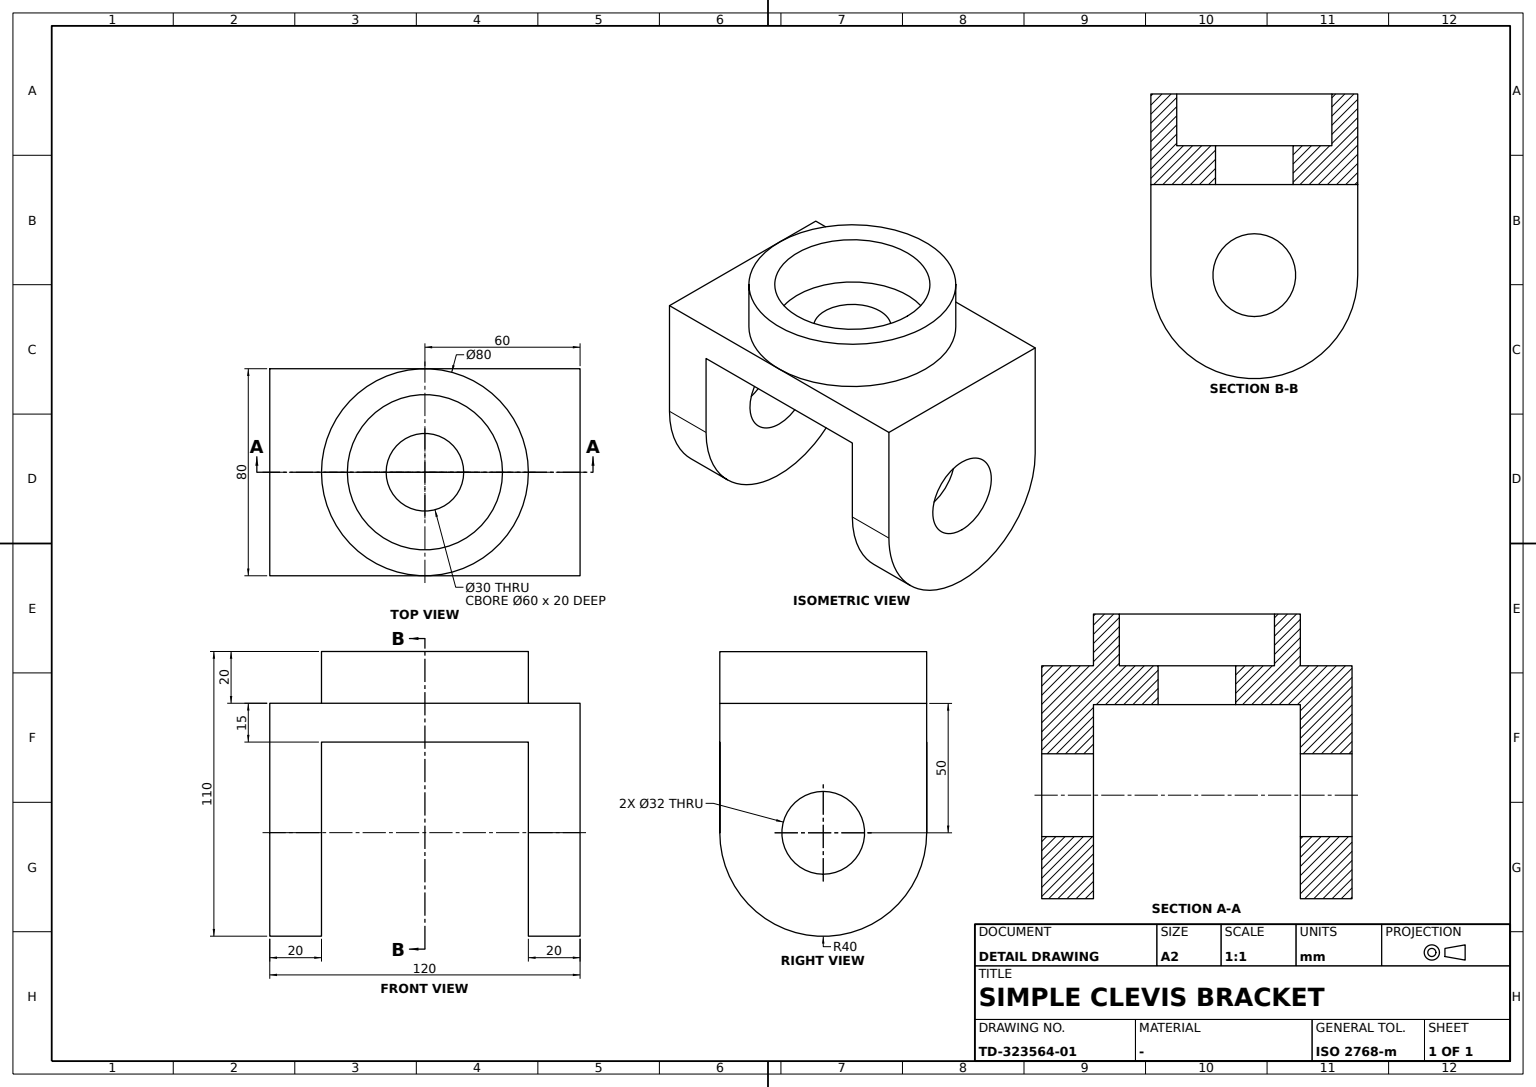
ISO-10303-21;
HEADER;
FILE_DESCRIPTION((''),'2;1');
FILE_NAME('','',(''),(''),'','','');
FILE_SCHEMA(('AUTOMOTIVE_DESIGN'));
ENDSEC;
DATA;
#1=APPLICATION_CONTEXT('');
#2=PRODUCT_CONTEXT('',#1,'mechanical');
#3=PRODUCT('','','',(#2));
#4=PRODUCT_DEFINITION_FORMATION('','',#3);
#5=PRODUCT_DEFINITION_CONTEXT('',#1,'design');
#6=PRODUCT_DEFINITION('','',#4,#5);
#7=PRODUCT_DEFINITION_SHAPE('','',#6);
#8=(LENGTH_UNIT()NAMED_UNIT(*)SI_UNIT(.MILLI.,.METRE.));
#9=(NAMED_UNIT(*)PLANE_ANGLE_UNIT()SI_UNIT($,.RADIAN.));
#10=(NAMED_UNIT(*)SI_UNIT($,.STERADIAN.)SOLID_ANGLE_UNIT());
#11=UNCERTAINTY_MEASURE_WITH_UNIT(LENGTH_MEASURE(0.005),#8,'distance_accuracy_value','');
#12=(GEOMETRIC_REPRESENTATION_CONTEXT(3)GLOBAL_UNCERTAINTY_ASSIGNED_CONTEXT((#11))GLOBAL_UNIT_ASSIGNED_CONTEXT((#8,#9,#10))REPRESENTATION_CONTEXT('',''));
#13=CARTESIAN_POINT('',(-40.,0.,-51.));
#14=VERTEX_POINT('',#13);
#15=CARTESIAN_POINT('',(-40.,0.,-35.));
#16=DIRECTION('',(1.,0.,0.));
#17=DIRECTION('',(0.,0.,-1.));
#18=AXIS2_PLACEMENT_3D('',#15,#16,#17);
#19=CIRCLE('',#18,16.);
#20=EDGE_CURVE('',#14,#14,#19,.T.);
#21=ORIENTED_EDGE('',*,*,#20,.T.);
#22=EDGE_LOOP('',(#21));
#23=FACE_BOUND('',#22,.T.);
#24=CARTESIAN_POINT('',(-60.,0.,-51.));
#25=VERTEX_POINT('',#24);
#26=CARTESIAN_POINT('',(-60.,0.,-35.));
#27=AXIS2_PLACEMENT_3D('',#26,#16,#17);
#28=CIRCLE('',#27,16.);
#29=EDGE_CURVE('',#25,#25,#28,.T.);
#30=ORIENTED_EDGE('',*,*,#29,.F.);
#31=EDGE_LOOP('',(#30));
#32=FACE_BOUND('',#31,.T.);
#33=CARTESIAN_POINT('',(50.,0.,-35.));
#34=DIRECTION('',(0.,1.,0.));
#35=AXIS2_PLACEMENT_3D('',#33,#16,#34);
#36=CYLINDRICAL_SURFACE('',#35,16.);
#37=ADVANCED_FACE('',(#23,#32),#36,.F.);
#38=CARTESIAN_POINT('',(60.,0.,-19.));
#39=VERTEX_POINT('',#38);
#40=CARTESIAN_POINT('',(60.,0.,-35.));
#41=DIRECTION('',(-1.,0.,0.));
#42=DIRECTION('',(0.,0.,1.));
#43=AXIS2_PLACEMENT_3D('',#40,#41,#42);
#44=CIRCLE('',#43,16.);
#45=EDGE_CURVE('',#39,#39,#44,.F.);
#46=ORIENTED_EDGE('',*,*,#45,.F.);
#47=EDGE_LOOP('',(#46));
#48=FACE_BOUND('',#47,.T.);
#49=CARTESIAN_POINT('',(60.,-40.,-35.));
#50=VERTEX_POINT('',#49);
#51=CARTESIAN_POINT('',(60.,40.,-35.));
#52=VERTEX_POINT('',#51);
#53=CIRCLE('',#43,40.);
#54=EDGE_CURVE('',#50,#52,#53,.F.);
#55=ORIENTED_EDGE('',*,*,#54,.T.);
#56=CARTESIAN_POINT('',(60.,40.,15.));
#57=VERTEX_POINT('',#56);
#58=CARTESIAN_POINT('',(60.,40.,0.));
#59=VECTOR('',#42,1000.);
#60=LINE('',#58,#59);
#61=EDGE_CURVE('',#52,#57,#60,.T.);
#62=ORIENTED_EDGE('',*,*,#61,.T.);
#63=CARTESIAN_POINT('',(60.,-40.,15.));
#64=VERTEX_POINT('',#63);
#65=VECTOR('',#34,1000.);
#66=LINE('',#56,#65);
#67=EDGE_CURVE('',#64,#57,#66,.T.);
#68=ORIENTED_EDGE('',*,*,#67,.F.);
#69=CARTESIAN_POINT('',(60.,-40.,0.));
#70=VECTOR('',#17,1000.);
#71=LINE('',#69,#70);
#72=EDGE_CURVE('',#64,#50,#71,.T.);
#73=ORIENTED_EDGE('',*,*,#72,.T.);
#74=EDGE_LOOP('',(#55,#62,#68,#73));
#75=FACE_BOUND('',#74,.T.);
#76=DIRECTION('',(0.,-1.,0.));
#77=AXIS2_PLACEMENT_3D('',#58,#41,#76);
#78=PLANE('',#77);
#79=ADVANCED_FACE('',(#48,#75),#78,.F.);
#80=CARTESIAN_POINT('',(40.,40.,0.));
#81=VERTEX_POINT('',#80);
#82=CARTESIAN_POINT('',(40.,-40.,0.));
#83=VERTEX_POINT('',#82);
#84=CARTESIAN_POINT('',(40.,0.,0.));
#85=VECTOR('',#76,1000.);
#86=LINE('',#84,#85);
#87=EDGE_CURVE('',#81,#83,#86,.T.);
#88=ORIENTED_EDGE('',*,*,#87,.F.);
#89=CARTESIAN_POINT('',(40.,40.,-35.));
#90=VERTEX_POINT('',#89);
#91=LINE('',#80,#59);
#92=EDGE_CURVE('',#90,#81,#91,.T.);
#93=ORIENTED_EDGE('',*,*,#92,.F.);
#94=CARTESIAN_POINT('',(40.,-40.,-35.));
#95=VERTEX_POINT('',#94);
#96=CARTESIAN_POINT('',(40.,0.,-35.));
#97=AXIS2_PLACEMENT_3D('',#96,#16,#17);
#98=CIRCLE('',#97,40.);
#99=EDGE_CURVE('',#95,#90,#98,.T.);
#100=ORIENTED_EDGE('',*,*,#99,.F.);
#101=LINE('',#82,#70);
#102=EDGE_CURVE('',#83,#95,#101,.T.);
#103=ORIENTED_EDGE('',*,*,#102,.F.);
#104=EDGE_LOOP('',(#88,#93,#100,#103));
#105=FACE_BOUND('',#104,.T.);
#106=CARTESIAN_POINT('',(40.,0.,-51.));
#107=VERTEX_POINT('',#106);
#108=CIRCLE('',#97,16.);
#109=EDGE_CURVE('',#107,#107,#108,.T.);
#110=ORIENTED_EDGE('',*,*,#109,.T.);
#111=EDGE_LOOP('',(#110));
#112=FACE_BOUND('',#111,.T.);
#113=AXIS2_PLACEMENT_3D('',#84,#16,#34);
#114=PLANE('',#113);
#115=ADVANCED_FACE('',(#105,#112),#114,.F.);
#116=CARTESIAN_POINT('',(15.,0.,0.));
#117=VERTEX_POINT('',#116);
#118=CARTESIAN_POINT('',(0.,0.,0.));
#119=AXIS2_PLACEMENT_3D('',#118,#42,#16);
#120=CIRCLE('',#119,15.);
#121=EDGE_CURVE('',#117,#117,#120,.T.);
#122=ORIENTED_EDGE('',*,*,#121,.T.);
#123=EDGE_LOOP('',(#122));
#124=FACE_BOUND('',#123,.T.);
#125=CARTESIAN_POINT('',(-40.,40.,0.));
#126=VERTEX_POINT('',#125);
#127=CARTESIAN_POINT('',(-40.,-40.,0.));
#128=VERTEX_POINT('',#127);
#129=CARTESIAN_POINT('',(-40.,0.,0.));
#130=LINE('',#129,#85);
#131=EDGE_CURVE('',#126,#128,#130,.T.);
#132=ORIENTED_EDGE('',*,*,#131,.F.);
#133=CARTESIAN_POINT('',(0.,40.,0.));
#134=VECTOR('',#16,1000.);
#135=LINE('',#133,#134);
#136=EDGE_CURVE('',#126,#81,#135,.T.);
#137=ORIENTED_EDGE('',*,*,#136,.T.);
#138=ORIENTED_EDGE('',*,*,#87,.T.);
#139=CARTESIAN_POINT('',(0.,-40.,0.));
#140=VECTOR('',#41,1000.);
#141=LINE('',#139,#140);
#142=EDGE_CURVE('',#83,#128,#141,.T.);
#143=ORIENTED_EDGE('',*,*,#142,.T.);
#144=EDGE_LOOP('',(#132,#137,#138,#143));
#145=FACE_BOUND('',#144,.T.);
#146=PLANE('',#119);
#147=ADVANCED_FACE('',(#124,#145),#146,.F.);
#148=ORIENTED_EDGE('',*,*,#54,.F.);
#149=CARTESIAN_POINT('',(50.,-40.,-35.));
#150=LINE('',#149,#134);
#151=EDGE_CURVE('',#50,#95,#150,.F.);
#152=ORIENTED_EDGE('',*,*,#151,.T.);
#153=ORIENTED_EDGE('',*,*,#99,.T.);
#154=CARTESIAN_POINT('',(50.,40.,-35.));
#155=LINE('',#154,#134);
#156=EDGE_CURVE('',#52,#90,#155,.F.);
#157=ORIENTED_EDGE('',*,*,#156,.F.);
#158=EDGE_LOOP('',(#148,#152,#153,#157));
#159=FACE_BOUND('',#158,.T.);
#160=CYLINDRICAL_SURFACE('',#35,40.);
#161=ADVANCED_FACE('',(#159),#160,.T.);
#162=CARTESIAN_POINT('',(-60.,-40.,15.));
#163=VERTEX_POINT('',#162);
#164=CARTESIAN_POINT('',(-60.,-40.,-35.));
#165=VERTEX_POINT('',#164);
#166=CARTESIAN_POINT('',(-60.,-40.,0.));
#167=LINE('',#166,#70);
#168=EDGE_CURVE('',#163,#165,#167,.T.);
#169=ORIENTED_EDGE('',*,*,#168,.T.);
#170=CARTESIAN_POINT('',(-40.,-40.,-35.));
#171=VERTEX_POINT('',#170);
#172=EDGE_CURVE('',#165,#171,#150,.T.);
#173=ORIENTED_EDGE('',*,*,#172,.T.);
#174=LINE('',#127,#70);
#175=EDGE_CURVE('',#128,#171,#174,.T.);
#176=ORIENTED_EDGE('',*,*,#175,.F.);
#177=ORIENTED_EDGE('',*,*,#142,.F.);
#178=ORIENTED_EDGE('',*,*,#102,.T.);
#179=ORIENTED_EDGE('',*,*,#151,.F.);
#180=ORIENTED_EDGE('',*,*,#72,.F.);
#181=CARTESIAN_POINT('',(0.,-40.,15.));
#182=VERTEX_POINT('',#181);
#183=LINE('',#181,#140);
#184=EDGE_CURVE('',#64,#182,#183,.T.);
#185=ORIENTED_EDGE('',*,*,#184,.T.);
#186=LINE('',#63,#134);
#187=EDGE_CURVE('',#163,#182,#186,.T.);
#188=ORIENTED_EDGE('',*,*,#187,.F.);
#189=EDGE_LOOP('',(#169,#173,#176,#177,#178,#179,#180,#185,#188));
#190=FACE_BOUND('',#189,.T.);
#191=AXIS2_PLACEMENT_3D('',#69,#34,#41);
#192=PLANE('',#191);
#193=ADVANCED_FACE('',(#190),#192,.F.);
#194=CARTESIAN_POINT('',(15.,0.,15.));
#195=VERTEX_POINT('',#194);
#196=CARTESIAN_POINT('',(0.,0.,15.));
#197=AXIS2_PLACEMENT_3D('',#196,#42,#16);
#198=CIRCLE('',#197,15.);
#199=EDGE_CURVE('',#195,#195,#198,.T.);
#200=ORIENTED_EDGE('',*,*,#199,.F.);
#201=EDGE_LOOP('',(#200));
#202=FACE_BOUND('',#201,.T.);
#203=CARTESIAN_POINT('',(30.,0.,15.));
#204=VERTEX_POINT('',#203);
#205=CIRCLE('',#197,30.);
#206=EDGE_CURVE('',#204,#204,#205,.T.);
#207=ORIENTED_EDGE('',*,*,#206,.T.);
#208=EDGE_LOOP('',(#207));
#209=FACE_BOUND('',#208,.T.);
#210=PLANE('',#197);
#211=ADVANCED_FACE('',(#202,#209),#210,.T.);
#212=ORIENTED_EDGE('',*,*,#206,.F.);
#213=EDGE_LOOP('',(#212));
#214=FACE_BOUND('',#213,.T.);
#215=CARTESIAN_POINT('',(30.,0.,35.));
#216=VERTEX_POINT('',#215);
#217=CARTESIAN_POINT('',(0.,0.,35.));
#218=AXIS2_PLACEMENT_3D('',#217,#42,#16);
#219=CIRCLE('',#218,30.);
#220=EDGE_CURVE('',#216,#216,#219,.T.);
#221=ORIENTED_EDGE('',*,*,#220,.T.);
#222=EDGE_LOOP('',(#221));
#223=FACE_BOUND('',#222,.T.);
#224=CARTESIAN_POINT('',(0.,0.,25.));
#225=AXIS2_PLACEMENT_3D('',#224,#42,#16);
#226=CYLINDRICAL_SURFACE('',#225,30.);
#227=ADVANCED_FACE('',(#214,#223),#226,.F.);
#228=ORIENTED_EDGE('',*,*,#20,.F.);
#229=EDGE_LOOP('',(#228));
#230=FACE_BOUND('',#229,.T.);
#231=CARTESIAN_POINT('',(-40.,40.,-35.));
#232=VERTEX_POINT('',#231);
#233=CIRCLE('',#18,40.);
#234=EDGE_CURVE('',#171,#232,#233,.T.);
#235=ORIENTED_EDGE('',*,*,#234,.T.);
#236=LINE('',#125,#59);
#237=EDGE_CURVE('',#232,#126,#236,.T.);
#238=ORIENTED_EDGE('',*,*,#237,.T.);
#239=ORIENTED_EDGE('',*,*,#131,.T.);
#240=ORIENTED_EDGE('',*,*,#175,.T.);
#241=EDGE_LOOP('',(#235,#238,#239,#240));
#242=FACE_BOUND('',#241,.T.);
#243=AXIS2_PLACEMENT_3D('',#129,#16,#34);
#244=PLANE('',#243);
#245=ADVANCED_FACE('',(#230,#242),#244,.T.);
#246=ORIENTED_EDGE('',*,*,#29,.T.);
#247=EDGE_LOOP('',(#246));
#248=FACE_BOUND('',#247,.T.);
#249=CARTESIAN_POINT('',(-60.,40.,-35.));
#250=VERTEX_POINT('',#249);
#251=CARTESIAN_POINT('',(-60.,40.,15.));
#252=VERTEX_POINT('',#251);
#253=CARTESIAN_POINT('',(-60.,40.,0.));
#254=LINE('',#253,#59);
#255=EDGE_CURVE('',#250,#252,#254,.T.);
#256=ORIENTED_EDGE('',*,*,#255,.F.);
#257=CIRCLE('',#27,40.);
#258=EDGE_CURVE('',#165,#250,#257,.T.);
#259=ORIENTED_EDGE('',*,*,#258,.F.);
#260=ORIENTED_EDGE('',*,*,#168,.F.);
#261=CARTESIAN_POINT('',(-60.,0.,15.));
#262=LINE('',#261,#65);
#263=EDGE_CURVE('',#163,#252,#262,.T.);
#264=ORIENTED_EDGE('',*,*,#263,.T.);
#265=EDGE_LOOP('',(#256,#259,#260,#264));
#266=FACE_BOUND('',#265,.T.);
#267=AXIS2_PLACEMENT_3D('',#166,#16,#34);
#268=PLANE('',#267);
#269=ADVANCED_FACE('',(#248,#266),#268,.F.);
#270=ORIENTED_EDGE('',*,*,#258,.T.);
#271=EDGE_CURVE('',#250,#232,#155,.T.);
#272=ORIENTED_EDGE('',*,*,#271,.T.);
#273=ORIENTED_EDGE('',*,*,#234,.F.);
#274=ORIENTED_EDGE('',*,*,#172,.F.);
#275=EDGE_LOOP('',(#270,#272,#273,#274));
#276=FACE_BOUND('',#275,.T.);
#277=ADVANCED_FACE('',(#276),#160,.T.);
#278=CARTESIAN_POINT('',(40.,0.,35.));
#279=VERTEX_POINT('',#278);
#280=CIRCLE('',#218,40.);
#281=EDGE_CURVE('',#279,#279,#280,.T.);
#282=ORIENTED_EDGE('',*,*,#281,.F.);
#283=EDGE_LOOP('',(#282));
#284=FACE_BOUND('',#283,.T.);
#285=CARTESIAN_POINT('',(0.,40.,15.));
#286=VERTEX_POINT('',#285);
#287=CIRCLE('',#197,40.);
#288=EDGE_CURVE('',#286,#182,#287,.T.);
#289=ORIENTED_EDGE('',*,*,#288,.T.);
#290=EDGE_CURVE('',#182,#286,#287,.T.);
#291=ORIENTED_EDGE('',*,*,#290,.T.);
#292=EDGE_LOOP('',(#289,#291));
#293=FACE_BOUND('',#292,.T.);
#294=CYLINDRICAL_SURFACE('',#225,40.);
#295=ADVANCED_FACE('',(#284,#293),#294,.T.);
#296=ORIENTED_EDGE('',*,*,#237,.F.);
#297=ORIENTED_EDGE('',*,*,#271,.F.);
#298=ORIENTED_EDGE('',*,*,#255,.T.);
#299=LINE('',#285,#134);
#300=EDGE_CURVE('',#252,#286,#299,.T.);
#301=ORIENTED_EDGE('',*,*,#300,.T.);
#302=EDGE_CURVE('',#286,#57,#299,.T.);
#303=ORIENTED_EDGE('',*,*,#302,.T.);
#304=ORIENTED_EDGE('',*,*,#61,.F.);
#305=ORIENTED_EDGE('',*,*,#156,.T.);
#306=ORIENTED_EDGE('',*,*,#92,.T.);
#307=ORIENTED_EDGE('',*,*,#136,.F.);
#308=EDGE_LOOP('',(#296,#297,#298,#301,#303,#304,#305,#306,#307));
#309=FACE_BOUND('',#308,.T.);
#310=AXIS2_PLACEMENT_3D('',#253,#76,#16);
#311=PLANE('',#310);
#312=ADVANCED_FACE('',(#309),#311,.F.);
#313=ORIENTED_EDGE('',*,*,#121,.F.);
#314=EDGE_LOOP('',(#313));
#315=FACE_BOUND('',#314,.T.);
#316=ORIENTED_EDGE('',*,*,#199,.T.);
#317=EDGE_LOOP('',(#316));
#318=FACE_BOUND('',#317,.T.);
#319=CARTESIAN_POINT('',(0.,0.,5.));
#320=AXIS2_PLACEMENT_3D('',#319,#42,#16);
#321=CYLINDRICAL_SURFACE('',#320,15.);
#322=ADVANCED_FACE('',(#315,#318),#321,.F.);
#323=ORIENTED_EDGE('',*,*,#281,.T.);
#324=EDGE_LOOP('',(#323));
#325=FACE_BOUND('',#324,.T.);
#326=ORIENTED_EDGE('',*,*,#220,.F.);
#327=EDGE_LOOP('',(#326));
#328=FACE_BOUND('',#327,.T.);
#329=PLANE('',#218);
#330=ADVANCED_FACE('',(#325,#328),#329,.T.);
#331=ORIENTED_EDGE('',*,*,#300,.F.);
#332=ORIENTED_EDGE('',*,*,#263,.F.);
#333=ORIENTED_EDGE('',*,*,#187,.T.);
#334=ORIENTED_EDGE('',*,*,#288,.F.);
#335=EDGE_LOOP('',(#331,#332,#333,#334));
#336=FACE_BOUND('',#335,.T.);
#337=ADVANCED_FACE('',(#336),#210,.T.);
#338=ORIENTED_EDGE('',*,*,#45,.T.);
#339=EDGE_LOOP('',(#338));
#340=FACE_BOUND('',#339,.T.);
#341=ORIENTED_EDGE('',*,*,#109,.F.);
#342=EDGE_LOOP('',(#341));
#343=FACE_BOUND('',#342,.T.);
#344=ADVANCED_FACE('',(#340,#343),#36,.F.);
#345=ORIENTED_EDGE('',*,*,#184,.F.);
#346=ORIENTED_EDGE('',*,*,#67,.T.);
#347=ORIENTED_EDGE('',*,*,#302,.F.);
#348=ORIENTED_EDGE('',*,*,#290,.F.);
#349=EDGE_LOOP('',(#345,#346,#347,#348));
#350=FACE_BOUND('',#349,.T.);
#351=ADVANCED_FACE('',(#350),#210,.T.);
#352=CLOSED_SHELL('',(#37,#79,#115,#147,#161,#193,#211,#227,#245,#269,#277,#295,#312,#322,#330,#337,#344,#351));
#353=MANIFOLD_SOLID_BREP('',#352);
#354=ADVANCED_BREP_SHAPE_REPRESENTATION('',(#353),#12);
#355=SHAPE_DEFINITION_REPRESENTATION(#7,#354);
ENDSEC;
END-ISO-10303-21;
